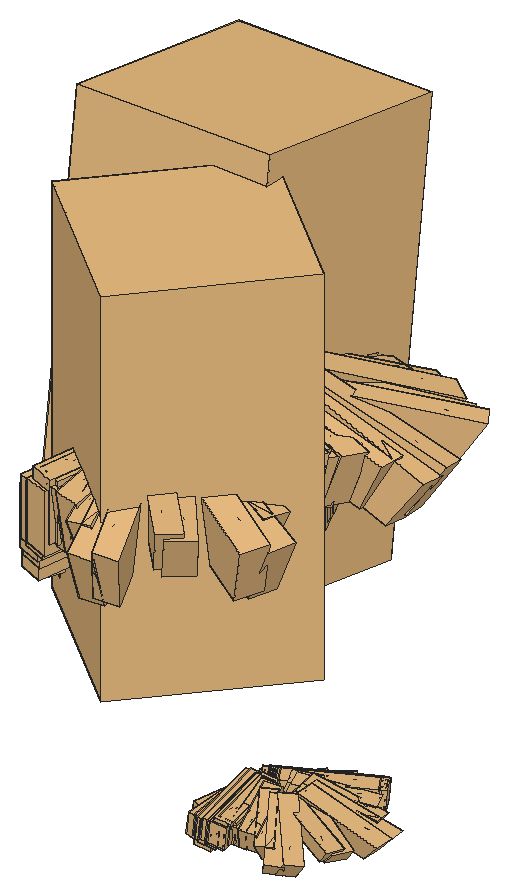
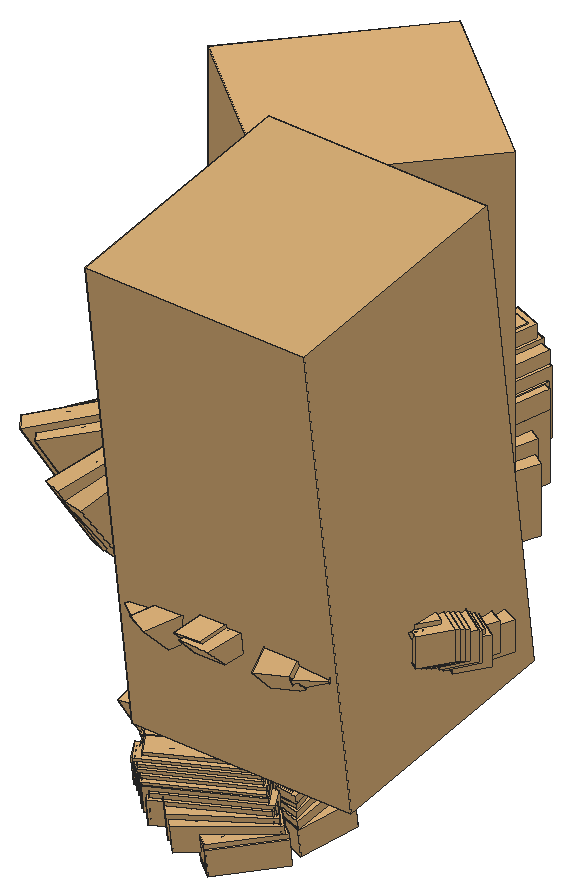
# SketchUp Ruby script. Lengths in inches.
U = 1.inch
M = Sketchup.active_model
def pt(a) = Geom::Point3d.new(a.map { |v| v * U })
def face(e, loops, mat)
  f = e.add_face(loops[0].map { |a| pt(a) })
  loops[1..].each { |l| e.add_face(l.map { |a| pt(a) }).erase! }
  f.material = f.back_material = mat if mat
  f
end
# faces: each face lists its corners as indices into pts; further lists are holes
def faces(e, pts, list, mat = nil) = list.each { |f| face(e, (f[0].is_a?(Array) ? f : [f]).map { |l| l.map { |i| pts[i] } }, mat) }
# xy, xz, yz: faces in a plane at the given z, y or x. An outline is a flat list of corners, or four numbers for a rectangle; further outlines are holes
def ring(l) = l.size == 4 ? [[l[0], l[1]], [l[2], l[1]], [l[2], l[3]], [l[0], l[3]]] : l.each_slice(2).to_a
def flat(e, list, mat, &to3) = list.each { |f| face(e, (f[0].is_a?(Array) ? f : [f]).map { |l| ring(l).map { |u, v| to3.(u, v) } }, mat) }
def xy(e, z, list, mat = nil) = flat(e, list, mat) { |x, y| [x, y, z] }
def xz(e, y, list, mat = nil) = flat(e, list, mat) { |x, z| [x, y, z] }
def yz(e, x, list, mat = nil) = flat(e, list, mat) { |y, z| [x, y, z] }
def lines(e, pts, list) = list.each { |a, b| e.add_line(pt(pts[a]), pt(pts[b])) }
# prism: a flat outline (further loops are holes) pulled along v
def prism(e, loops, v, mat = nil)
  f = face(e, loops, mat); d = Geom::Vector3d.new(v.map { |x| x * U })
  f.pushpull(f.normal.samedirection?(d) ? d.length : -d.length)
end
def box(e, o, s, mat = nil) = prism(e, [[o, [o[0] + s[0], o[1], o[2]], [o[0] + s[0], o[1] + s[1], o[2]], [o[0], o[1] + s[1], o[2]]]], [0, 0, s[2]], mat)
def at(x, y, z, deg = 0) = Geom::Transformation.translation(pt([x, y, z])) * Geom::Transformation.rotation(ORIGIN, Z_AXIS, deg.degrees)
def axes(o, x, y, z) = Geom::Transformation.new([*x, 0, *y, 0, *z, 0, *pt(o).to_a, 1])
def part(name) = M.definitions.add(name)
# library, detail: a bought-in or finely detailed component or shape, given as its bounding box
def library(name, o, s) = part(name).tap { |d| box(d.entities, o, s) }
def detail(e, o, s) = box(e.add_group.entities, o, s)
def put(e, d, t, mat = nil) = e.add_instance(d, t).tap { |i| i.material = mat if mat }
def group(e, t, mat = nil) = e.add_group.tap { |g| g.transformation = t; g.material = mat if mat }.entities
root = M.entities
M.materials.add("AM85_043_stem").color = [137, 75, 57]
c1 = part("Leaf blade")
p = [[83.87,1.9,45.32],[93.74,4.15,37.73],[37.05,-3.5625,61.7],[49.38,-2.58,60.05],[69.4,9.27,54.68],[74.7,9.96,52.16],
  [102.49,6.87,29.18],[110.02,10.09,19.93],[45.83,5.6,61.35],[51.45,6.53,60.35],[91.18,12.19,41.53],[94.56,12.64,38.66],
  [12.82,-5.2,59.53],[24.77,-4.41,61.53],[22.59,0.63,61.46],[34.04,3.3,62.19],[61.47,-1.4,56.68],[73.04,0.08,51.71],
  [109.02,14.97,22.84],[115.89,16.47,11.9375]]
lines(c1.entities,p,[[0,1],[2,3],[4,5],[6,7],[8,9],[10,11],[12,13],[14,15],[16,17],[18,19]])
detail(c1.entities,[1.52,-6.02,0.37],[119.64,24.16,61.82])
c2 = part("Group\#250")
p = [[69.397,177.044,-76.908],[69.056,177.22,-76.772],[69.397,177.397,-76.635],[69.739,177.22,-76.772],[69.397,126.923,-36.489],[68.124,127.405,-35.832],
  [69.397,153.661,-55.129],[70.671,127.405,-35.832],[68.59,154.026,-54.756],[70.205,154.026,-54.756],[69.397,127.887,-35.175],[69.397,154.392,-54.384],
  [69.397,97.5,-21.509],[67.658,98.015,-20.533],[71.137,98.015,-20.533],[69.397,98.53,-19.558],[69.397,66.147,-10.6],[67.192,66.605,-9.289],
  [71.603,66.605,-9.289],[69.397,67.064,-7.977],[69.397,33.682,-4.048],[66.726,33.994,-2.4],[72.069,33.994,-2.4],[69.397,34.304,-0.752],
  [69.397,0.958,-2],[66.26,1.035,-0.035],[69.397,1.112,1.931],[72.535,1.035,-0.035],[69.397,0.956,-2]]
faces(c2.entities,p,[[0,1,2,3]])
faces(c2.entities,p,[[4,5,6],[4,6,7],[8,6,5],[9,7,6],[5,10,11,8],[7,9,11,10],[12,13,4],[12,4,14],
  [5,4,13],[7,14,4],[13,15,10,5],[14,7,10,15],[16,17,12],[16,12,18],[13,12,17],[14,18,12],
  [17,19,15,13],[18,14,15,19],[16,20,17],[16,18,20],[21,17,20],[22,20,18],[21,23,17],[22,18,23],
  [19,17,23],[19,23,18],[20,24,21],[20,22,24],[25,21,24],[25,26,21],[27,24,22],[22,23,27],
  [23,21,26],[28,25,24],[28,27,25],[28,24,27],[26,27,23],[26,25,27]],"AM85_043_stem")
c3 = library("Group\#251",[25.96,5.88,-22.96],[170.77,196.24,312.95])
c4 = library("Group\#253",[26.16,5.88,-22.96],[170.57,196.24,312.95])
g1 = group(root,at(460.25,63.92,66.36))
put(g1,c1,axes([1.79,16.1,12.08],[0.08905,-0.07244,0.00538],[0.08172,0.11708,0.00062],[-0.01512,0.01001,0.0496]))
put(g1,c1,axes([0.3125,14.91,12.48],[0.10261,-0.0691,0],[0.07204,0.12425,0],[0,0,0.05002]))
put(g1,c1,axes([26.59,14.41,11.73],[-0.09758,-0.07764,0],[-0.06098,0.12425,0],[0,0,0.05002]))
put(g1,c1,axes([2.36,1.5625,7.29],[0.08954,-0.02156,0],[0.02257,0.14383,0],[0,0,0.05002]))
put(g1,c1,axes([12.45,28.89,13.55],[-0.00474,-0.13925,0.00237],[0.13587,-0.00486,0.00008],[0,0.03607,0.03572]))
put(g1,c1,axes([-0.95,10.6,10.15],[0.11529,-0.07764,0],[0.07204,0.12425,0],[0,0,0.05002]))
put(g1,c1,axes([-0.48,5.65,8.6],[0.11114,-0.05011,0],[0.04045,0.13768,0],[0,0,0.05002]))
put(g1,c1,axes([2.38,1.86,7.75],[0.08954,-0.02156,0],[0.02257,0.14383,0],[0,0,0.05002]))
put(g1,c1,axes([-1.53,10.375,9.67],[0.11529,-0.07764,0],[0.07204,0.12425,0],[0,0,0.05002]))
put(g1,c1,axes([24.04,16.25,12.02],[-0.07537,-0.07244,0.00538],[-0.06917,0.11708,0.00062],[0.01279,0.01001,0.0496]))
put(g1,c1,axes([2.94,17.8125,12.2],[0.07973,-0.07758,0.00659],[0.09082,0.109,0.00081],[-0.01809,0.01436,0.04934]))
put(g1,c1,axes([-1.53,11.61,10.55],[0.11529,-0.07764,0],[0.07204,0.12425,0],[0,0,0.05002]))
put(g1,c1,axes([20.81,26.42,11.91],[-0.04503,-0.12644,0.01599],[-0.10576,0.0562,-0.0045],[0.00518,0.0482,0.04719]))
put(g1,c1,axes([22.02,24.64,11.52],[-0.05563,-0.11649,0.01832],[-0.09826,0.07625,0.00012],[0.02216,0.04566,0.04655]))
put(g1,c1,axes([26.85,11.76,10.49],[-0.09758,-0.07764,0],[-0.06098,0.12425,0],[0,0,0.05002]))
put(g1,c1,axes([26.85,10.71,10.49],[-0.09758,-0.07764,0],[-0.06098,0.12425,0],[0,0,0.05002]))
put(g1,c1,axes([27.15,12.51,11.01],[-0.09758,-0.07764,0],[-0.06098,0.12425,0],[0,0,0.05002]))
put(g1,c1,axes([-1.53,12.12,10.86],[0.11529,-0.07764,0],[0.07204,0.12425,0],[0,0,0.05002]))
put(g1,c1,axes([4.18,24.49,11.57],[0.06573,-0.11649,0.01832],[0.11609,0.07625,0.00012],[-0.02618,0.04566,0.04655]))
put(g1,c1,axes([15.02,28.4,13.8125],[0.00402,-0.13925,0.00237],[-0.115,-0.00486,0.00008],[0,0.03607,0.03572]))
put(g1,c1,axes([25.96,5.8,8.54],[-0.09407,-0.05011,0],[-0.03424,0.13768,0],[0,0,0.05002]))
put(g1,c1,axes([23.54,2.02,7.7],[-0.07579,-0.02156,0],[-0.0191,0.14383,0],[0,0,0.05002]))
put(g1,c1,axes([26.85,10.53,9.61],[-0.09758,-0.07764,0],[-0.06098,0.12425,0],[0,0,0.05002]))
put(g1,c1,axes([26.07,14.53,12.3],[-0.08685,-0.0691,0],[-0.06098,0.12425,0],[0,0,0.05002]))
put(g1,c1,axes([26.7,13.85,11.4375],[-0.09758,-0.07764,0],[-0.06098,0.12425,0],[0,0,0.05002]))
put(g1,c1,axes([-1.23,13.55,11.48],[0.11529,-0.07764,0],[0.07204,0.12425,0],[0,0,0.05002]))
put(g1,c1,axes([-1.23,14.94,12.08],[0.11529,-0.07764,0],[0.07204,0.12425,0],[0,0,0.05002]))
put(g1,c1,axes([5.61,26.26,11.96],[0.05321,-0.12644,0.01599],[0.12496,0.0562,-0.0045],[-0.00612,0.0482,0.04719]))
put(g1,c1,axes([-1.23,14.25,11.79],[0.11529,-0.07764,0],[0.07204,0.12425,0],[0,0,0.05002]))
put(g1,c1,axes([-1.23,12.86,11.18],[0.11529,-0.07764,0],[0.07204,0.12425,0],[0,0,0.05002]))
put(g1,c1,axes([25.29,14.7,12.3],[-0.08685,-0.0691,0],[-0.06098,0.12425,0],[0,0,0.05002]))
put(g1,c1,axes([5.35,21.6,12],[0.05777,-0.0989,0.01148],[0.10937,0.08305,0.00887],[-0.04092,0.01929,0.04725]))
put(g1,c1,axes([23.07,17.96,12.14],[-0.06748,-0.07758,0.00659],[-0.07687,0.109,0.00081],[0.01531,0.01436,0.04934]))
put(g1,c1,axes([-0.26,7.49,9.19],[0.10805,-0.05959,0],[0.04811,0.13385,0],[0,0,0.05002]))
put(g1,c1,axes([27.04,12.95,11.56],[-0.09758,-0.07764,0],[-0.06098,0.12425,0],[0,0,0.05002]))
put(g1,c1,axes([21.03,21.75,11.94],[-0.0489,-0.0989,0.01148],[-0.09257,0.08305,0.00887],[0.03464,0.01929,0.04725]))
put(g1,c1,axes([25.77,7.64,9.14],[-0.09145,-0.05959,0],[-0.04072,0.13385,0],[0,0,0.05002]))
put(g1,c2,axes([2.46,1.12,7.21],[0.16801,0,0],[0,0.01889,0.046],[0,-0.14378,0.00861]))
put(root,c3,axes([458.08,63.39,74.64],[0.13801,0.00021,0.0027],[0.00019,0.12586,-0.01977],[-0.00301,0.02391,0.15213]))
put(root,c4,axes([483.21,78.27,74.9],[-0.08104,-0.09786,0],[0.09033,-0.07479,0],[0,0,0.14177]))
g2 = group(root,at(465.92,75.61,77.5))
put(g2,c1,axes([13.67,9.66,7.47],[-0.00424,-0.10647,0.02015],[0.13249,0.00074,-0.02131],[0.01708,0.02455,0.10296]))
put(g2,c1,axes([12.11,10.21,8.5625],[0.00369,-0.11587,0.0078],[0.13241,0.01194,-0.02345],[0.0179,0.00764,0.10498]))
put(g2,c1,axes([25.71,-10.3,6.11],[-0.11123,0.03279,0.01659],[0.06031,0.11378,-0.01857],[0.0179,0.00764,0.10498]))
put(g2,c1,axes([1.34,0.64,-0.17],[0.03233,-0.08019,0.00032],[0.1203,0.06038,-0.02491],[0.0179,0.00764,0.10498]))
put(g2,c1,axes([29.59,8.63,8.02],[-0.10635,-0.0712,0.02847],[0.07002,-0.10663,-0.004],[0.03989,0.02493,0.06892]))
put(g2,c1,axes([7.36,8.49,4.4375],[0.00415,-0.13019,0.00877],[0.13241,0.01194,-0.02345],[0.0179,0.00764,0.10498]))
put(g2,c1,axes([3.34,5.22,1.99],[0.02259,-0.11215,0.00431],[0.12538,0.04337,-0.02454],[0.0179,0.00764,0.10498]))
put(g2,c1,axes([1.75,0.86,0.75],[0.03233,-0.08019,0.00032],[0.1203,0.06038,-0.02491],[0.0179,0.00764,0.10498]))
put(g2,c1,axes([6.7,8.74,3.49],[0.00415,-0.13019,0.00877],[0.13241,0.01194,-0.02345],[0.0179,0.00764,0.10498]))
put(g2,c1,axes([25.82,-7.3,6.51],[-0.09336,0.01941,0.02619],[0.0507,0.11627,-0.01577],[0.03221,0.00318,0.10193]))
put(g2,c1,axes([15.62,9.72,7.39],[-0.01272,-0.10192,0.02389],[0.13142,-0.01055,-0.01989],[0.01865,0.02914,0.10179]))
put(g2,c1,axes([7.95,9.55,5.14],[0.00415,-0.13019,0.00877],[0.13241,0.01194,-0.02345],[0.0179,0.00764,0.10498]))
put(g2,c1,axes([31.67,0.64,4.68],[-0.11369,-0.03135,0.05638],[-0.01671,0.11063,-0.01497],[0.05591,0.02927,0.09076]))
put(g2,c1,axes([30.85,-1.3,4.11],[-0.11112,-0.01751,0.06],[0.00408,0.11642,-0.00891],[0.06298,0.0148,0.08922]))
put(g2,c1,axes([23.43,-12.11,3.95],[-0.11123,0.03279,0.01659],[0.06031,0.11378,-0.01857],[0.0179,0.00764,0.10498]))
put(g2,c1,axes([22.64,-12.68,4.125],[-0.11123,0.03279,0.01659],[0.06031,0.11378,-0.01857],[0.0179,0.00764,0.10498]))
put(g2,c1,axes([24.33,-11.86,4.9],[-0.11123,0.03279,0.01659],[0.06031,0.11378,-0.01857],[0.0179,0.00764,0.10498]))
put(g2,c1,axes([8.44,9.87,5.69],[0.00415,-0.13019,0.00877],[0.13241,0.01194,-0.02345],[0.0179,0.00764,0.10498]))
put(g2,c1,axes([21.09,12.28,4.92],[-0.04534,-0.11042,0.05555],[0.12026,-0.04769,-0.01678],[0.03678,0.05181,0.09099]))
put(g2,c1,axes([32.27,7.27,8.23],[-0.10161,-0.0779,0.02814],[-0.06595,0.08543,0.00521],[0.03989,0.02493,0.06892]))
put(g2,c1,axes([17.76,-14.95,0.88],[-0.08864,0.04496,0.01185],[0.08489,0.10056,-0.0218],[0.0179,0.00764,0.10498]))
put(g2,c1,axes([13.3,-15.26,-0.17],[-0.05728,0.04638,0.00639],[0.09772,0.09229,-0.02338],[0.0179,0.00764,0.10498]))
put(g2,c1,axes([22.18,-12.91,2.3],[-0.11123,0.03279,0.01659],[0.06031,0.11378,-0.01857],[0.0179,0.00764,0.10498]))
put(g2,c1,axes([25.73,-9.75,7.3125],[-0.099,0.02918,0.01476],[0.06031,0.11378,-0.01857],[0.0179,0.00764,0.10498]))
put(g2,c1,axes([25.25,-10.72,5.58],[-0.11123,0.03279,0.01659],[0.06031,0.11378,-0.01857],[0.0179,0.00764,0.10498]))
put(g2,c1,axes([9.9,10.5,6.75],[0.00415,-0.13019,0.00877],[0.13241,0.01194,-0.02345],[0.0179,0.00764,0.10498]))
put(g2,c1,axes([11.17,11.34,7.79],[0.00415,-0.13019,0.00877],[0.13241,0.01194,-0.02345],[0.0179,0.00764,0.10498]))
put(g2,c1,axes([23.33,12.21,5.39],[-0.06044,-0.10657,0.05277],[0.10834,-0.06601,-0.02344],[0.04979,0.03791,0.09118]))
put(g2,c1,axes([10.54,10.93,7.27],[0.00415,-0.13019,0.00877],[0.13241,0.01194,-0.02345],[0.0179,0.00764,0.10498]))
put(g2,c1,axes([9.27,10.08,6.23],[0.00415,-0.13019,0.00877],[0.13241,0.01194,-0.02345],[0.0179,0.00764,0.10498]))
put(g2,c1,axes([25.43,-9.06,7.3125],[-0.099,0.02918,0.01476],[0.06031,0.11378,-0.01857],[0.0179,0.00764,0.10498]))
put(g2,c1,axes([19.7,9.89,6.25],[-0.03889,-0.09588,0.03854],[0.12486,-0.03754,0.0007],[0.00923,0.04896,0.09742]))
put(g2,c1,axes([26.625,-5.61,6.51],[-0.09251,0.01078,0.0293],[0.04053,0.11783,-0.01373],[0.03675,0.00357,0.10057]))
put(g2,c1,axes([5.05,6.14,2.93],[0.01379,-0.1149,0.00601],[0.12665,0.03544,-0.02418],[0.0179,0.00764,0.10498]))
put(g2,c1,axes([24.8,-11.46,5.98],[-0.11123,0.03279,0.01659],[0.06031,0.11378,-0.01857],[0.0179,0.00764,0.10498]))
put(g2,c1,axes([28.29,-2.04,5.53],[-0.09671,-0.01421,0.04245],[0.0154,0.11708,0.00811],[0.05018,-0.00889,0.09465]))
put(g2,c1,axes([19.26,-13.72,1.83],[-0.09435,0.03784,0.01334],[0.0785,0.10345,-0.02092],[0.0179,0.00764,0.10498]))
put(g2,c2,axes([1.03,0.32,-0.26],[0.09106,-0.12863,-0.00617],[0.03065,0.01722,0.09337],[-0.10495,-0.07632,0.04215]))
g3 = group(root,at(482.9375,73.74,73.55))
put(g3,c1,axes([11.11,-11.64,10.98],[-0.11442,-0.00685,0.0122],[0.01918,-0.14133,0.0014],[0.01787,0.00285,0.11252]))
put(g3,c1,axes([11.39,-9.77,11.88],[-0.12212,-0.01846,0],[0.03115,-0.14008,0],[0,0,0.11349]))
put(g3,c1,axes([-8.25,-27.15,10.18],[0.01915,0.12303,0],[0.12885,-0.05023,0],[0,0,0.11349]))
put(g3,c1,axes([0.86,-1.34,0.11],[-0.08036,-0.04461,0],[0.08073,-0.12106,0],[0,0,0.11349]))
put(g3,c1,axes([11.93,-28.26,14.32],[-0.09072,0.10566,0.00538],[-0.10309,-0.08819,0.00019],[0.0244,-0.02654,0.08104]))
put(g3,c1,axes([9.4,-5.75,6.6],[-0.13721,-0.02075,0],[0.03115,-0.14008,0],[0,0,0.11349]))
put(g3,c1,axes([5.7,-2.42,3.08],[-0.11554,-0.0382,0],[0.06343,-0.12862,0],[0,0,0.11349]))
put(g3,c1,axes([1.04,-1.57,1.16],[-0.08036,-0.04461,0],[0.08073,-0.12106,0],[0,0,0.11349]))
put(g3,c1,axes([9.68,-5.1875,5.51],[-0.13721,-0.02075,0],[0.03115,-0.14008,0],[0,0,0.11349]))
put(g3,c1,axes([-5.13,-26.78,10.85],[0.00635,0.10421,0.0122],[0.13001,-0.03942,0.0014],[-0.00263,-0.01601,0.11252]))
put(g3,c1,axes([11.42,-13.68,11.25],[-0.11104,0.00323,0.01495],[0.00703,-0.14154,0.00184],[0.023,0.00165,0.11193]))
put(g3,c1,axes([10.51,-6.1,7.51],[-0.13721,-0.02075,0],[0.03115,-0.14008,0],[0,0,0.11349]))
put(g3,c1,axes([4.12,-32.08,10.59],[-0.05246,0.12344,0.03627],[0.1157,0.03009,-0.0102],[0.0288,-0.03896,0.10705]))
put(g3,c1,axes([2.03,-31.59,9.7],[-0.03794,0.12328,0.04157],[0.12376,0.01027,0.00027],[0.01462,-0.04856,0.1056]))
put(g3,c1,axes([-10.23,-25.38,7.38],[0.01915,0.12303,0],[0.12885,-0.05023,0],[0,0,0.11349]))
put(g3,c1,axes([-10.94,-24.61,7.38],[0.01915,0.12303,0],[0.12885,-0.05023,0],[0,0,0.11349]))
put(g3,c1,axes([-9.94,-26.13,8.5625],[0.01915,0.12303,0],[0.12885,-0.05023,0],[0,0,0.11349]))
put(g3,c1,axes([10.86,-6.47,8.2],[-0.13721,-0.02075,0],[0.03115,-0.14008,0],[0,0,0.11349]))
put(g3,c1,axes([15.03,-19.43,9.83],[-0.12709,0.04131,0.04157],[-0.03368,-0.13451,0.00027],[0.05012,-0.01591,0.1056]))
put(g3,c1,axes([9.72,-29.63,14.91],[-0.09716,0.09974,0.00538],[0.08118,0.08125,0.00019],[0.0244,-0.02654,0.08104]))
put(g3,c1,axes([-13.61,-20.39,2.95],[0.03519,0.10041,0],[0.1183,-0.07817,0],[0,0,0.11349]))
put(g3,c1,axes([-14.39,-15.97,1.03],[0.04108,0.06705,0],[0.11133,-0.09292,0],[0,0,0.11349]))
put(g3,c1,axes([-11.07,-24.47,5.38],[0.01915,0.12303,0],[0.12885,-0.05023,0],[0,0,0.11349]))
put(g3,c1,axes([-7.79,-26.89,11.49],[0.01704,0.1095,0],[0.12885,-0.05023,0],[0,0,0.11349]))
put(g3,c1,axes([-8.71,-26.82,9.52],[0.01915,0.12303,0],[0.12885,-0.05023,0],[0,0,0.11349]))
put(g3,c1,axes([11.6,-7.73,9.62],[-0.13721,-0.02075,0],[0.03115,-0.14008,0],[0,0,0.11349]))
put(g3,c1,axes([12.54,-8.76,10.99],[-0.13721,-0.02075,0],[0.03115,-0.14008,0],[0,0,0.11349]))
put(g3,c1,axes([15.18,-21.7,10.72],[-0.12462,0.05709,0.03627],[-0.05376,-0.12574,-0.0102],[0.0371,-0.03133,0.10705]))
put(g3,c1,axes([12.08,-8.25,10.3125],[-0.13721,-0.02075,0],[0.03115,-0.14008,0],[0,0,0.11349]))
put(g3,c1,axes([11.13,-7.22,8.93],[-0.13721,-0.02075,0],[0.03115,-0.14008,0],[0,0,0.11349]))
put(g3,c1,axes([-7.1,-26.49,11.49],[0.01704,0.1095,0],[0.12885,-0.05023,0],[0,0,0.11349]))
put(g3,c1,axes([12.22,-18.09,10.79],[-0.10934,0.03374,0.02605],[-0.02415,-0.13498,0.02013],[0.04311,0.01345,0.10719]))
put(g3,c1,axes([-3.26,-27.39,11.12],[-0.00292,0.10265,0.01495],[0.13021,-0.02828,0.00184],[-0.00153,-0.02091,0.11193]))
put(g3,c1,axes([6.79,-3.93,4.43],[-0.11968,-0.02913,0],[0.05522,-0.13097,0],[0,0,0.11349]))
put(g3,c1,axes([-9.57,-26.38,9.8],[0.01915,0.12303,0],[0.12885,-0.05023,0],[0,0,0.11349]))
put(g3,c1,axes([0.8,-28.8,10.66],[-0.03099,0.10579,0.02605],[0.12418,0.00142,0.02013],[-0.01239,-0.03759,0.10719]))
put(g3,c1,axes([-12.23,-21.62,4.3],[0.02686,0.10562,0],[0.12046,-0.07098,0],[0,0,0.11349]))
put(g3,c2,axes([0.49,-1.08,-0.0625],[-0.1234,-0.11348,0],[0.01278,-0.01389,0.10435],[-0.09727,0.10579,0.01954]))
g4 = group(root,at(485.8125,78.67,41.8))
put(g4,c1,axes([11.1,-7.47,9.97],[-0.0707,-0.02736,0.00376],[0.05469,-0.09852,0.00545],[0.01495,0.00596,0.03888]))
put(g4,c1,axes([10.75,-6.06,10.22],[-0.07262,-0.03732,-0.0001],[0.06192,-0.09527,0.00499],[0.0044,0.0004,0.0392]))
put(g4,c1,axes([3.33,-22.5,10.11],[-0.02462,0.0928,-0.00411],[0.09752,-0.01108,0.0025],[0.0044,0.0004,0.0392]))
put(g4,c1,axes([1.03,-2.0625,5.8],[-0.03806,-0.04805,0.00105],[0.08795,-0.07178,0.00464],[0.0044,0.0004,0.0392]))
put(g4,c1,axes([16.74,-19.32,11.7],[-0.08952,0.05869,-0.00231],[-0.03954,-0.08405,0.00247],[0.02671,-0.01414,0.02905]))
put(g4,c1,axes([8.07,-3.56,8.25],[-0.0816,-0.04193,-0.00011],[0.06192,-0.09527,0.00499],[0.0044,0.0004,0.0392]))
put(g4,c1,axes([4.57,-1.89,6.89],[-0.0625,-0.05031,0.00061],[0.07915,-0.08065,0.00479],[0.0044,0.0004,0.0392]))
put(g4,c1,axes([1.26,-2.19,6.17],[-0.03806,-0.04805,0.00105],[0.08795,-0.07178,0.00464],[0.0044,0.0004,0.0392]))
put(g4,c1,axes([8.04,-3.1,7.85],[-0.0816,-0.04193,-0.00011],[0.06192,-0.09527,0.00499],[0.0044,0.0004,0.0392]))
put(g4,c1,axes([5.24,-21.61,10.35],[-0.02669,0.07671,0.00068],[0.09508,-0.00302,0.00262],[0.00748,-0.0117,0.0394]))
put(g4,c1,axes([11.93,-8.89,10.14],[-0.07145,-0.01939,0.00438],[0.04699,-0.10105,0.00553],[0.01857,0.0061,0.03874]))
put(g4,c1,axes([8.93,-3.59,8.58],[-0.0816,-0.04193,-0.00011],[0.06192,-0.09527,0.00499],[0.0044,0.0004,0.0392]))
put(g4,c1,axes([12.74,-23.64,10.5],[-0.06916,0.07918,0.00798],[0.06464,0.04443,-0.00386],[0.03426,-0.02217,0.03849]))
put(g4,c1,axes([11.22,-23.69,10.16],[-0.05962,0.08193,0.0099],[0.07614,0.03171,0.00049],[0.028,-0.03191,0.03823]))
put(g4,c1,axes([1.42,-21.61,9.07],[-0.02462,0.0928,-0.00411],[0.09752,-0.01108,0.0025],[0.0044,0.0004,0.0392]))
put(g4,c1,axes([0.74,-21.19,9.04],[-0.02462,0.0928,-0.00411],[0.09752,-0.01108,0.0025],[0.0044,0.0004,0.0392]))
put(g4,c1,axes([1.88,-22.1,9.51],[-0.02462,0.0928,-0.00411],[0.09752,-0.01108,0.0025],[0.0044,0.0004,0.0392]))
put(g4,c1,axes([9.29,-3.79,8.83],[-0.0816,-0.04193,-0.00011],[0.06192,-0.09527,0.00499],[0.0044,0.0004,0.0392]))
put(g4,c1,axes([15.9,-12.35,9.87],[-0.0921,0.00512,0.01218],[0.01877,-0.10396,0.00451],[0.04094,-0.00132,0.03732]))
put(g4,c1,axes([15.76,-20.75,11.9375],[-0.09186,0.05315,-0.00215],[0.02761,0.07473,-0.00223],[0.02671,-0.01414,0.02905]))
put(g4,c1,axes([-2.41,-18.68,7.35],[-0.00757,0.07957,-0.00323],[0.09914,-0.03337,0.00339],[0.0044,0.0004,0.0392]))
put(g4,c1,axes([-4.31,-15.64,6.53],[0.0062,0.05659,-0.00205],[0.0991,-0.04541,0.00386],[0.0044,0.0004,0.0392]))
put(g4,c1,axes([0.54,-21.125,8.34],[-0.02462,0.0928,-0.00411],[0.09752,-0.01108,0.0025],[0.0044,0.0004,0.0392]))
put(g4,c1,axes([3.6,-22.21,10.56],[-0.02191,0.08259,-0.00365],[0.09752,-0.01108,0.0025],[0.0044,0.0004,0.0392]))
put(g4,c1,axes([2.91,-22.35,9.87],[-0.02462,0.0928,-0.00411],[0.09752,-0.01108,0.0025],[0.0044,0.0004,0.0392]))
put(g4,c1,axes([10.19,-4.55,9.37],[-0.0816,-0.04193,-0.00011],[0.06192,-0.09527,0.00499],[0.0044,0.0004,0.0392]))
put(g4,c1,axes([11.16,-5.1,9.88],[-0.0816,-0.04193,-0.00011],[0.06192,-0.09527,0.00499],[0.0044,0.0004,0.0392]))
put(g4,c1,axes([16.71,-13.95,10.25],[-0.09546,0.017,0.00982],[0.00288,-0.10159,0.00046],[0.03728,-0.01502,0.03828]))
put(g4,c1,axes([10.68,-4.83,9.63],[-0.0816,-0.04193,-0.00011],[0.06192,-0.09527,0.00499],[0.0044,0.0004,0.0392]))
put(g4,c1,axes([9.71,-4.27,9.11],[-0.0816,-0.04193,-0.00011],[0.06192,-0.09527,0.00499],[0.0044,0.0004,0.0392]))
put(g4,c1,axes([3.92,-21.78,10.55],[-0.02191,0.08259,-0.00365],[0.09752,-0.01108,0.0025],[0.0044,0.0004,0.0392]))
put(g4,c1,axes([13.74,-11.92,10.14],[-0.07908,0.00307,0.00718],[0.02578,-0.10235,0.01144],[0.02772,0.01856,0.03682]))
put(g4,c1,axes([6.63,-21.68,10.47],[-0.03205,0.07378,0.00162],[0.09188,0.00508,0.00239],[0.00963,-0.01504,0.03937]))
put(g4,c1,axes([5.77,-2.76,7.42],[-0.06786,-0.04456,0.00028],[0.07459,-0.08396,0.00483],[0.0044,0.0004,0.0392]))
put(g4,c1,axes([2.24,-22.2,9.94],[-0.02462,0.0928,-0.00411],[0.09752,-0.01108,0.0025],[0.0044,0.0004,0.0392]))
put(g4,c1,axes([9.64,-21.91,10.39],[-0.05053,0.07058,0.00518],[0.07983,0.02546,0.00765],[0.00749,-0.02926,0.03824]))
put(g4,c1,axes([-1.1,-19.29,7.87],[-0.01447,0.08171,-0.00346],[0.09837,-0.02774,0.00316],[0.0044,0.0004,0.0392]))
put(g4,c2,axes([0.71,-1.95,5.73],[-0.04497,-0.10633,0.00315],[0.01639,-0.00718,0.0366],[-0.0932,0.05755,0.00253]))
